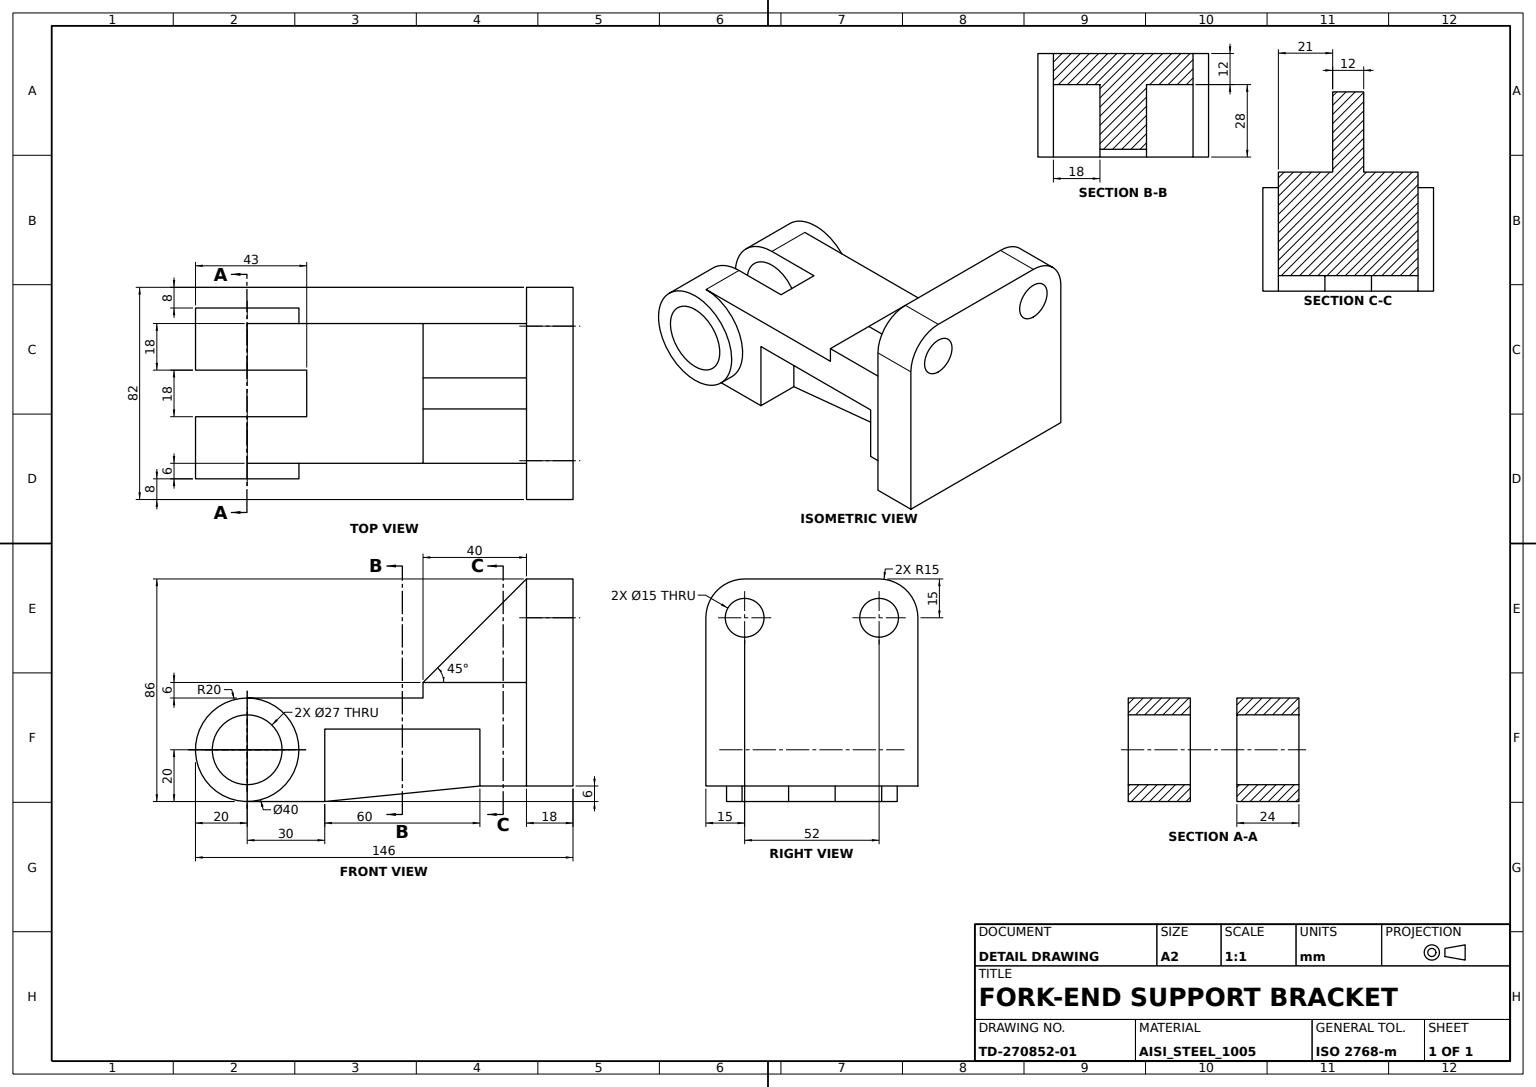
ISO-10303-21;
HEADER;
FILE_DESCRIPTION((''),'2;1');
FILE_NAME('','',(''),(''),'','','');
FILE_SCHEMA(('AUTOMOTIVE_DESIGN'));
ENDSEC;
DATA;
#1=APPLICATION_CONTEXT('');
#2=PRODUCT_CONTEXT('',#1,'mechanical');
#3=PRODUCT('','','',(#2));
#4=PRODUCT_DEFINITION_FORMATION('','',#3);
#5=PRODUCT_DEFINITION_CONTEXT('',#1,'design');
#6=PRODUCT_DEFINITION('','',#4,#5);
#7=PRODUCT_DEFINITION_SHAPE('','',#6);
#8=(LENGTH_UNIT()NAMED_UNIT(*)SI_UNIT(.MILLI.,.METRE.));
#9=(NAMED_UNIT(*)PLANE_ANGLE_UNIT()SI_UNIT($,.RADIAN.));
#10=(NAMED_UNIT(*)SI_UNIT($,.STERADIAN.)SOLID_ANGLE_UNIT());
#11=UNCERTAINTY_MEASURE_WITH_UNIT(LENGTH_MEASURE(0.005),#8,'distance_accuracy_value','');
#12=(GEOMETRIC_REPRESENTATION_CONTEXT(3)GLOBAL_UNCERTAINTY_ASSIGNED_CONTEXT((#11))GLOBAL_UNIT_ASSIGNED_CONTEXT((#8,#9,#10))REPRESENTATION_CONTEXT('',''));
#13=CARTESIAN_POINT('',(9.,-96.,-46.));
#14=VERTEX_POINT('',#13);
#15=CARTESIAN_POINT('',(-9.,-96.,-46.));
#16=VERTEX_POINT('',#15);
#17=DIRECTION('',(-1.,0.,0.));
#18=VECTOR('',#17,1000.);
#19=LINE('',#13,#18);
#20=EDGE_CURVE('',#14,#16,#19,.T.);
#21=ORIENTED_EDGE('',*,*,#20,.F.);
#22=CARTESIAN_POINT('',(27.,-96.,-46.));
#23=VERTEX_POINT('',#22);
#24=LINE('',#22,#18);
#25=EDGE_CURVE('',#23,#14,#24,.T.);
#26=ORIENTED_EDGE('',*,*,#25,.F.);
#27=CARTESIAN_POINT('',(27.,-126.,-46.));
#28=VERTEX_POINT('',#27);
#29=DIRECTION('',(0.,1.,0.));
#30=VECTOR('',#29,1000.);
#31=LINE('',#27,#30);
#32=EDGE_CURVE('',#28,#23,#31,.T.);
#33=ORIENTED_EDGE('',*,*,#32,.F.);
#34=CARTESIAN_POINT('',(9.,-126.,-46.));
#35=VERTEX_POINT('',#34);
#36=LINE('',#27,#18);
#37=EDGE_CURVE('',#28,#35,#36,.T.);
#38=ORIENTED_EDGE('',*,*,#37,.T.);
#39=CARTESIAN_POINT('',(9.,-103.,-46.));
#40=VERTEX_POINT('',#39);
#41=DIRECTION('',(0.,-1.,0.));
#42=VECTOR('',#41,1000.);
#43=LINE('',#34,#42);
#44=EDGE_CURVE('',#40,#35,#43,.T.);
#45=ORIENTED_EDGE('',*,*,#44,.F.);
#46=CARTESIAN_POINT('',(-9.,-103.,-46.));
#47=VERTEX_POINT('',#46);
#48=CARTESIAN_POINT('',(27.,-103.,-46.));
#49=DIRECTION('',(1.,0.,0.));
#50=VECTOR('',#49,1000.);
#51=LINE('',#48,#50);
#52=EDGE_CURVE('',#47,#40,#51,.T.);
#53=ORIENTED_EDGE('',*,*,#52,.F.);
#54=CARTESIAN_POINT('',(-9.,-126.,-46.));
#55=VERTEX_POINT('',#54);
#56=LINE('',#54,#30);
#57=EDGE_CURVE('',#55,#47,#56,.T.);
#58=ORIENTED_EDGE('',*,*,#57,.F.);
#59=CARTESIAN_POINT('',(-27.,-126.,-46.));
#60=VERTEX_POINT('',#59);
#61=EDGE_CURVE('',#55,#60,#36,.T.);
#62=ORIENTED_EDGE('',*,*,#61,.T.);
#63=CARTESIAN_POINT('',(-27.,-96.,-46.));
#64=VERTEX_POINT('',#63);
#65=LINE('',#59,#30);
#66=EDGE_CURVE('',#60,#64,#65,.T.);
#67=ORIENTED_EDGE('',*,*,#66,.T.);
#68=EDGE_CURVE('',#16,#64,#24,.T.);
#69=ORIENTED_EDGE('',*,*,#68,.F.);
#70=EDGE_LOOP('',(#21,#26,#33,#38,#45,#53,#58,#62,#67,#69));
#71=FACE_BOUND('',#70,.T.);
#72=DIRECTION('',(0.,0.,1.));
#73=AXIS2_PLACEMENT_3D('',#27,#72,#41);
#74=PLANE('',#73);
#75=ADVANCED_FACE('',(#71),#74,.F.);
#76=CARTESIAN_POINT('',(-6.,-18.,40.));
#77=VERTEX_POINT('',#76);
#78=CARTESIAN_POINT('',(-6.,-18.,0.));
#79=VERTEX_POINT('',#78);
#80=DIRECTION('',(0.,0.,-1.));
#81=VECTOR('',#80,1000.);
#82=LINE('',#76,#81);
#83=EDGE_CURVE('',#77,#79,#82,.T.);
#84=ORIENTED_EDGE('',*,*,#83,.T.);
#85=CARTESIAN_POINT('',(-6.,-58.,0.));
#86=VERTEX_POINT('',#85);
#87=LINE('',#78,#42);
#88=EDGE_CURVE('',#79,#86,#87,.T.);
#89=ORIENTED_EDGE('',*,*,#88,.T.);
#90=DIRECTION('',(0.,0.707106781,0.707106781));
#91=VECTOR('',#90,1000.);
#92=LINE('',#85,#91);
#93=EDGE_CURVE('',#86,#77,#92,.T.);
#94=ORIENTED_EDGE('',*,*,#93,.T.);
#95=EDGE_LOOP('',(#84,#89,#94));
#96=FACE_BOUND('',#95,.T.);
#97=CARTESIAN_POINT('',(-6.,0.,0.));
#98=AXIS2_PLACEMENT_3D('',#97,#17,#72);
#99=PLANE('',#98);
#100=ADVANCED_FACE('',(#96),#99,.T.);
#101=CARTESIAN_POINT('',(-9.,-36.,-18.));
#102=VERTEX_POINT('',#101);
#103=CARTESIAN_POINT('',(-9.,-36.,-40.));
#104=VERTEX_POINT('',#103);
#105=LINE('',#101,#81);
#106=EDGE_CURVE('',#102,#104,#105,.T.);
#107=ORIENTED_EDGE('',*,*,#106,.F.);
#108=CARTESIAN_POINT('',(-27.,-36.,-18.));
#109=VERTEX_POINT('',#108);
#110=CARTESIAN_POINT('',(47.,-36.,-18.));
#111=LINE('',#110,#18);
#112=EDGE_CURVE('',#109,#102,#111,.F.);
#113=ORIENTED_EDGE('',*,*,#112,.F.);
#114=CARTESIAN_POINT('',(-27.,-36.,-40.));
#115=VERTEX_POINT('',#114);
#116=CARTESIAN_POINT('',(-27.,-36.,0.));
#117=VECTOR('',#72,1000.);
#118=LINE('',#116,#117);
#119=EDGE_CURVE('',#115,#109,#118,.T.);
#120=ORIENTED_EDGE('',*,*,#119,.F.);
#121=CARTESIAN_POINT('',(27.,-36.,-40.));
#122=LINE('',#121,#18);
#123=EDGE_CURVE('',#104,#115,#122,.T.);
#124=ORIENTED_EDGE('',*,*,#123,.F.);
#125=EDGE_LOOP('',(#107,#113,#120,#124));
#126=FACE_BOUND('',#125,.T.);
#127=CARTESIAN_POINT('',(47.,-36.,-57.));
#128=AXIS2_PLACEMENT_3D('',#127,#41,#80);
#129=PLANE('',#128);
#130=ADVANCED_FACE('',(#126),#129,.T.);
#131=ORIENTED_EDGE('',*,*,#123,.T.);
#132=CARTESIAN_POINT('',(-27.,-18.,-40.));
#133=VERTEX_POINT('',#132);
#134=LINE('',#132,#42);
#135=EDGE_CURVE('',#133,#115,#134,.T.);
#136=ORIENTED_EDGE('',*,*,#135,.F.);
#137=CARTESIAN_POINT('',(-41.,-18.,-40.));
#138=VERTEX_POINT('',#137);
#139=LINE('',#137,#50);
#140=EDGE_CURVE('',#138,#133,#139,.T.);
#141=ORIENTED_EDGE('',*,*,#140,.F.);
#142=CARTESIAN_POINT('',(-41.,0.,-40.));
#143=VERTEX_POINT('',#142);
#144=LINE('',#137,#30);
#145=EDGE_CURVE('',#138,#143,#144,.T.);
#146=ORIENTED_EDGE('',*,*,#145,.T.);
#147=CARTESIAN_POINT('',(41.,0.,-40.));
#148=VERTEX_POINT('',#147);
#149=LINE('',#142,#50);
#150=EDGE_CURVE('',#143,#148,#149,.T.);
#151=ORIENTED_EDGE('',*,*,#150,.T.);
#152=CARTESIAN_POINT('',(41.,-18.,-40.));
#153=VERTEX_POINT('',#152);
#154=LINE('',#152,#30);
#155=EDGE_CURVE('',#153,#148,#154,.T.);
#156=ORIENTED_EDGE('',*,*,#155,.F.);
#157=CARTESIAN_POINT('',(27.,-18.,-40.));
#158=VERTEX_POINT('',#157);
#159=EDGE_CURVE('',#158,#153,#139,.T.);
#160=ORIENTED_EDGE('',*,*,#159,.F.);
#161=VERTEX_POINT('',#121);
#162=LINE('',#157,#42);
#163=EDGE_CURVE('',#158,#161,#162,.T.);
#164=ORIENTED_EDGE('',*,*,#163,.T.);
#165=CARTESIAN_POINT('',(9.,-36.,-40.));
#166=VERTEX_POINT('',#165);
#167=EDGE_CURVE('',#161,#166,#122,.T.);
#168=ORIENTED_EDGE('',*,*,#167,.T.);
#169=LINE('',#165,#18);
#170=EDGE_CURVE('',#166,#104,#169,.T.);
#171=ORIENTED_EDGE('',*,*,#170,.T.);
#172=EDGE_LOOP('',(#131,#136,#141,#146,#151,#156,#160,#164,#168,#171));
#173=FACE_BOUND('',#172,.T.);
#174=AXIS2_PLACEMENT_3D('',#157,#80,#29);
#175=PLANE('',#174);
#176=ADVANCED_FACE('',(#173),#175,.T.);
#177=ORIENTED_EDGE('',*,*,#37,.F.);
#178=CARTESIAN_POINT('',(27.,-126.,-6.));
#179=VERTEX_POINT('',#178);
#180=CARTESIAN_POINT('',(27.,-126.,-26.));
#181=AXIS2_PLACEMENT_3D('',#180,#17,#72);
#182=CIRCLE('',#181,20.);
#183=EDGE_CURVE('',#28,#179,#182,.F.);
#184=ORIENTED_EDGE('',*,*,#183,.T.);
#185=CARTESIAN_POINT('',(9.,-126.,-6.));
#186=VERTEX_POINT('',#185);
#187=LINE('',#178,#18);
#188=EDGE_CURVE('',#179,#186,#187,.T.);
#189=ORIENTED_EDGE('',*,*,#188,.T.);
#190=CARTESIAN_POINT('',(9.,-126.,-26.));
#191=AXIS2_PLACEMENT_3D('',#190,#17,#41);
#192=CIRCLE('',#191,20.);
#193=EDGE_CURVE('',#35,#186,#192,.T.);
#194=ORIENTED_EDGE('',*,*,#193,.F.);
#195=EDGE_LOOP('',(#177,#184,#189,#194));
#196=FACE_BOUND('',#195,.T.);
#197=CARTESIAN_POINT('',(33.,-106.,-26.));
#198=VERTEX_POINT('',#197);
#199=CARTESIAN_POINT('',(33.,-126.,-26.));
#200=AXIS2_PLACEMENT_3D('',#199,#49,#29);
#201=CIRCLE('',#200,20.);
#202=EDGE_CURVE('',#198,#198,#201,.T.);
#203=ORIENTED_EDGE('',*,*,#202,.F.);
#204=EDGE_LOOP('',(#203));
#205=FACE_BOUND('',#204,.T.);
#206=AXIS2_PLACEMENT_3D('',#199,#17,#72);
#207=CYLINDRICAL_SURFACE('',#206,20.);
#208=ADVANCED_FACE('',(#196,#205),#207,.T.);
#209=CARTESIAN_POINT('',(9.,-96.,-18.));
#210=VERTEX_POINT('',#209);
#211=LINE('',#13,#117);
#212=EDGE_CURVE('',#14,#210,#211,.T.);
#213=ORIENTED_EDGE('',*,*,#212,.F.);
#214=DIRECTION('',(0.,-0.99503719,-0.099503719));
#215=VECTOR('',#214,1000.);
#216=LINE('',#165,#215);
#217=EDGE_CURVE('',#166,#14,#216,.T.);
#218=ORIENTED_EDGE('',*,*,#217,.F.);
#219=CARTESIAN_POINT('',(9.,-36.,-18.));
#220=VERTEX_POINT('',#219);
#221=LINE('',#219,#81);
#222=EDGE_CURVE('',#220,#166,#221,.T.);
#223=ORIENTED_EDGE('',*,*,#222,.F.);
#224=LINE('',#209,#30);
#225=EDGE_CURVE('',#210,#220,#224,.T.);
#226=ORIENTED_EDGE('',*,*,#225,.F.);
#227=EDGE_LOOP('',(#213,#218,#223,#226));
#228=FACE_BOUND('',#227,.T.);
#229=CARTESIAN_POINT('',(9.,0.,0.));
#230=AXIS2_PLACEMENT_3D('',#229,#17,#72);
#231=PLANE('',#230);
#232=ADVANCED_FACE('',(#228),#231,.F.);
#233=CARTESIAN_POINT('',(-26.,-18.,32.5));
#234=VERTEX_POINT('',#233);
#235=CARTESIAN_POINT('',(-26.,-18.,25.));
#236=AXIS2_PLACEMENT_3D('',#235,#29,#72);
#237=CIRCLE('',#236,7.5);
#238=EDGE_CURVE('',#234,#234,#237,.T.);
#239=ORIENTED_EDGE('',*,*,#238,.T.);
#240=EDGE_LOOP('',(#239));
#241=FACE_BOUND('',#240,.T.);
#242=ORIENTED_EDGE('',*,*,#140,.T.);
#243=CARTESIAN_POINT('',(-27.,-18.,0.));
#244=VERTEX_POINT('',#243);
#245=LINE('',#243,#81);
#246=EDGE_CURVE('',#244,#133,#245,.T.);
#247=ORIENTED_EDGE('',*,*,#246,.F.);
#248=CARTESIAN_POINT('',(27.,-18.,0.));
#249=LINE('',#248,#18);
#250=EDGE_CURVE('',#79,#244,#249,.T.);
#251=ORIENTED_EDGE('',*,*,#250,.F.);
#252=ORIENTED_EDGE('',*,*,#83,.F.);
#253=CARTESIAN_POINT('',(-26.,-18.,40.));
#254=VERTEX_POINT('',#253);
#255=CARTESIAN_POINT('',(26.,-18.,40.));
#256=LINE('',#255,#18);
#257=EDGE_CURVE('',#77,#254,#256,.T.);
#258=ORIENTED_EDGE('',*,*,#257,.T.);
#259=CARTESIAN_POINT('',(-41.,-18.,25.));
#260=VERTEX_POINT('',#259);
#261=AXIS2_PLACEMENT_3D('',#235,#41,#49);
#262=CIRCLE('',#261,15.);
#263=EDGE_CURVE('',#254,#260,#262,.T.);
#264=ORIENTED_EDGE('',*,*,#263,.T.);
#265=LINE('',#259,#81);
#266=EDGE_CURVE('',#260,#138,#265,.T.);
#267=ORIENTED_EDGE('',*,*,#266,.T.);
#268=EDGE_LOOP('',(#242,#247,#251,#252,#258,#264,#267));
#269=FACE_BOUND('',#268,.T.);
#270=CARTESIAN_POINT('',(26.,-18.,25.));
#271=AXIS2_PLACEMENT_3D('',#270,#41,#80);
#272=PLANE('',#271);
#273=ADVANCED_FACE('',(#241,#269),#272,.T.);
#274=CARTESIAN_POINT('',(9.,-139.5,-26.));
#275=VERTEX_POINT('',#274);
#276=CIRCLE('',#191,13.5);
#277=EDGE_CURVE('',#275,#275,#276,.F.);
#278=ORIENTED_EDGE('',*,*,#277,.F.);
#279=EDGE_LOOP('',(#278));
#280=FACE_BOUND('',#279,.T.);
#281=CARTESIAN_POINT('',(33.,-126.,-12.5));
#282=VERTEX_POINT('',#281);
#283=CIRCLE('',#206,13.5);
#284=EDGE_CURVE('',#282,#282,#283,.T.);
#285=ORIENTED_EDGE('',*,*,#284,.F.);
#286=EDGE_LOOP('',(#285));
#287=FACE_BOUND('',#286,.T.);
#288=CYLINDRICAL_SURFACE('',#206,13.5);
#289=ADVANCED_FACE('',(#280,#287),#288,.F.);
#290=ORIENTED_EDGE('',*,*,#225,.T.);
#291=CARTESIAN_POINT('',(27.,-36.,-18.));
#292=VERTEX_POINT('',#291);
#293=EDGE_CURVE('',#220,#292,#111,.F.);
#294=ORIENTED_EDGE('',*,*,#293,.T.);
#295=CARTESIAN_POINT('',(27.,-96.,-18.));
#296=VERTEX_POINT('',#295);
#297=CARTESIAN_POINT('',(27.,0.,-18.));
#298=LINE('',#297,#42);
#299=EDGE_CURVE('',#292,#296,#298,.T.);
#300=ORIENTED_EDGE('',*,*,#299,.T.);
#301=CARTESIAN_POINT('',(47.,-96.,-18.));
#302=LINE('',#301,#18);
#303=EDGE_CURVE('',#210,#296,#302,.F.);
#304=ORIENTED_EDGE('',*,*,#303,.F.);
#305=EDGE_LOOP('',(#290,#294,#300,#304));
#306=FACE_BOUND('',#305,.T.);
#307=AXIS2_PLACEMENT_3D('',#110,#80,#29);
#308=PLANE('',#307);
#309=ADVANCED_FACE('',(#306),#308,.T.);
#310=ORIENTED_EDGE('',*,*,#263,.F.);
#311=CARTESIAN_POINT('',(-26.,0.,40.));
#312=VERTEX_POINT('',#311);
#313=LINE('',#253,#30);
#314=EDGE_CURVE('',#254,#312,#313,.T.);
#315=ORIENTED_EDGE('',*,*,#314,.T.);
#316=CARTESIAN_POINT('',(-41.,0.,25.));
#317=VERTEX_POINT('',#316);
#318=CARTESIAN_POINT('',(-26.,0.,25.));
#319=AXIS2_PLACEMENT_3D('',#318,#41,#49);
#320=CIRCLE('',#319,15.);
#321=EDGE_CURVE('',#312,#317,#320,.T.);
#322=ORIENTED_EDGE('',*,*,#321,.T.);
#323=LINE('',#259,#30);
#324=EDGE_CURVE('',#260,#317,#323,.T.);
#325=ORIENTED_EDGE('',*,*,#324,.F.);
#326=EDGE_LOOP('',(#310,#315,#322,#325));
#327=FACE_BOUND('',#326,.T.);
#328=CYLINDRICAL_SURFACE('',#236,15.);
#329=ADVANCED_FACE('',(#327),#328,.T.);
#330=ORIENTED_EDGE('',*,*,#20,.T.);
#331=LINE('',#103,#215);
#332=EDGE_CURVE('',#104,#16,#331,.T.);
#333=ORIENTED_EDGE('',*,*,#332,.F.);
#334=ORIENTED_EDGE('',*,*,#170,.F.);
#335=ORIENTED_EDGE('',*,*,#217,.T.);
#336=EDGE_LOOP('',(#330,#333,#334,#335));
#337=FACE_BOUND('',#336,.T.);
#338=DIRECTION('',(0.,0.099503719,-0.99503719));
#339=DIRECTION('',(0.,0.99503719,0.099503719));
#340=AXIS2_PLACEMENT_3D('',#165,#338,#339);
#341=PLANE('',#340);
#342=ADVANCED_FACE('',(#337),#341,.T.);
#343=CARTESIAN_POINT('',(-9.,-112.5,-26.));
#344=VERTEX_POINT('',#343);
#345=CARTESIAN_POINT('',(-9.,-126.,-26.));
#346=AXIS2_PLACEMENT_3D('',#345,#49,#29);
#347=CIRCLE('',#346,13.5);
#348=EDGE_CURVE('',#344,#344,#347,.F.);
#349=ORIENTED_EDGE('',*,*,#348,.F.);
#350=EDGE_LOOP('',(#349));
#351=FACE_BOUND('',#350,.T.);
#352=CARTESIAN_POINT('',(-33.,-126.,-39.5));
#353=VERTEX_POINT('',#352);
#354=CARTESIAN_POINT('',(-33.,-126.,-26.));
#355=AXIS2_PLACEMENT_3D('',#354,#49,#80);
#356=CIRCLE('',#355,13.5);
#357=EDGE_CURVE('',#353,#353,#356,.T.);
#358=ORIENTED_EDGE('',*,*,#357,.F.);
#359=EDGE_LOOP('',(#358));
#360=FACE_BOUND('',#359,.T.);
#361=ADVANCED_FACE('',(#351,#360),#288,.F.);
#362=ORIENTED_EDGE('',*,*,#357,.T.);
#363=EDGE_LOOP('',(#362));
#364=FACE_BOUND('',#363,.T.);
#365=CARTESIAN_POINT('',(-33.,-106.,-26.));
#366=VERTEX_POINT('',#365);
#367=AXIS2_PLACEMENT_3D('',#354,#49,#29);
#368=CIRCLE('',#367,20.);
#369=EDGE_CURVE('',#366,#366,#368,.T.);
#370=ORIENTED_EDGE('',*,*,#369,.F.);
#371=EDGE_LOOP('',(#370));
#372=FACE_BOUND('',#371,.T.);
#373=PLANE('',#355);
#374=ADVANCED_FACE('',(#364,#372),#373,.F.);
#375=ORIENTED_EDGE('',*,*,#183,.F.);
#376=ORIENTED_EDGE('',*,*,#32,.T.);
#377=CARTESIAN_POINT('',(27.,-96.,0.));
#378=LINE('',#377,#81);
#379=EDGE_CURVE('',#296,#23,#378,.T.);
#380=ORIENTED_EDGE('',*,*,#379,.F.);
#381=ORIENTED_EDGE('',*,*,#299,.F.);
#382=CARTESIAN_POINT('',(27.,-36.,0.));
#383=LINE('',#382,#117);
#384=EDGE_CURVE('',#161,#292,#383,.T.);
#385=ORIENTED_EDGE('',*,*,#384,.F.);
#386=ORIENTED_EDGE('',*,*,#163,.F.);
#387=VERTEX_POINT('',#248);
#388=LINE('',#248,#81);
#389=EDGE_CURVE('',#387,#158,#388,.T.);
#390=ORIENTED_EDGE('',*,*,#389,.F.);
#391=CARTESIAN_POINT('',(27.,-58.,0.));
#392=VERTEX_POINT('',#391);
#393=CARTESIAN_POINT('',(27.,-126.,0.));
#394=LINE('',#393,#30);
#395=EDGE_CURVE('',#392,#387,#394,.T.);
#396=ORIENTED_EDGE('',*,*,#395,.F.);
#397=CARTESIAN_POINT('',(27.,-58.,-6.));
#398=VERTEX_POINT('',#397);
#399=LINE('',#391,#117);
#400=EDGE_CURVE('',#398,#392,#399,.T.);
#401=ORIENTED_EDGE('',*,*,#400,.F.);
#402=CARTESIAN_POINT('',(27.,0.,-6.));
#403=LINE('',#402,#30);
#404=EDGE_CURVE('',#179,#398,#403,.T.);
#405=ORIENTED_EDGE('',*,*,#404,.F.);
#406=EDGE_LOOP('',(#375,#376,#380,#381,#385,#386,#390,#396,#401,#405));
#407=FACE_BOUND('',#406,.T.);
#408=CARTESIAN_POINT('',(27.,0.,0.));
#409=AXIS2_PLACEMENT_3D('',#408,#17,#72);
#410=PLANE('',#409);
#411=ADVANCED_FACE('',(#407),#410,.F.);
#412=ORIENTED_EDGE('',*,*,#52,.T.);
#413=CARTESIAN_POINT('',(9.,-103.,-6.));
#414=VERTEX_POINT('',#413);
#415=CARTESIAN_POINT('',(9.,-103.,34.));
#416=LINE('',#415,#81);
#417=EDGE_CURVE('',#40,#414,#416,.F.);
#418=ORIENTED_EDGE('',*,*,#417,.T.);
#419=CARTESIAN_POINT('',(-9.,-103.,-6.));
#420=VERTEX_POINT('',#419);
#421=CARTESIAN_POINT('',(47.,-103.,-6.));
#422=LINE('',#421,#50);
#423=EDGE_CURVE('',#420,#414,#422,.T.);
#424=ORIENTED_EDGE('',*,*,#423,.F.);
#425=CARTESIAN_POINT('',(-9.,-103.,34.));
#426=LINE('',#425,#81);
#427=EDGE_CURVE('',#47,#420,#426,.F.);
#428=ORIENTED_EDGE('',*,*,#427,.F.);
#429=EDGE_LOOP('',(#412,#418,#424,#428));
#430=FACE_BOUND('',#429,.T.);
#431=AXIS2_PLACEMENT_3D('',#415,#41,#80);
#432=PLANE('',#431);
#433=ADVANCED_FACE('',(#430),#432,.T.);
#434=CARTESIAN_POINT('',(-9.,-126.,-6.));
#435=VERTEX_POINT('',#434);
#436=CARTESIAN_POINT('',(-9.,-133.,-6.));
#437=LINE('',#436,#30);
#438=EDGE_CURVE('',#435,#420,#437,.T.);
#439=ORIENTED_EDGE('',*,*,#438,.F.);
#440=CIRCLE('',#346,20.);
#441=EDGE_CURVE('',#435,#55,#440,.T.);
#442=ORIENTED_EDGE('',*,*,#441,.T.);
#443=ORIENTED_EDGE('',*,*,#57,.T.);
#444=ORIENTED_EDGE('',*,*,#427,.T.);
#445=EDGE_LOOP('',(#439,#442,#443,#444));
#446=FACE_BOUND('',#445,.T.);
#447=ORIENTED_EDGE('',*,*,#348,.T.);
#448=EDGE_LOOP('',(#447));
#449=FACE_BOUND('',#448,.T.);
#450=AXIS2_PLACEMENT_3D('',#425,#49,#29);
#451=PLANE('',#450);
#452=ADVANCED_FACE('',(#446,#449),#451,.T.);
#453=ORIENTED_EDGE('',*,*,#238,.F.);
#454=EDGE_LOOP('',(#453));
#455=FACE_BOUND('',#454,.T.);
#456=CARTESIAN_POINT('',(-26.,0.,17.5));
#457=VERTEX_POINT('',#456);
#458=AXIS2_PLACEMENT_3D('',#318,#41,#80);
#459=CIRCLE('',#458,7.5);
#460=EDGE_CURVE('',#457,#457,#459,.T.);
#461=ORIENTED_EDGE('',*,*,#460,.F.);
#462=EDGE_LOOP('',(#461));
#463=FACE_BOUND('',#462,.T.);
#464=CYLINDRICAL_SURFACE('',#236,7.5);
#465=ADVANCED_FACE('',(#455,#463),#464,.F.);
#466=ORIENTED_EDGE('',*,*,#277,.T.);
#467=EDGE_LOOP('',(#466));
#468=FACE_BOUND('',#467,.T.);
#469=ORIENTED_EDGE('',*,*,#193,.T.);
#470=CARTESIAN_POINT('',(9.,-133.,-6.));
#471=LINE('',#470,#42);
#472=EDGE_CURVE('',#414,#186,#471,.T.);
#473=ORIENTED_EDGE('',*,*,#472,.F.);
#474=ORIENTED_EDGE('',*,*,#417,.F.);
#475=ORIENTED_EDGE('',*,*,#44,.T.);
#476=EDGE_LOOP('',(#469,#473,#474,#475));
#477=FACE_BOUND('',#476,.T.);
#478=CARTESIAN_POINT('',(9.,-183.,34.));
#479=AXIS2_PLACEMENT_3D('',#478,#17,#41);
#480=PLANE('',#479);
#481=ADVANCED_FACE('',(#468,#477),#480,.T.);
#482=ORIENTED_EDGE('',*,*,#93,.F.);
#483=CARTESIAN_POINT('',(6.,-58.,0.));
#484=VERTEX_POINT('',#483);
#485=LINE('',#483,#18);
#486=EDGE_CURVE('',#484,#86,#485,.T.);
#487=ORIENTED_EDGE('',*,*,#486,.F.);
#488=CARTESIAN_POINT('',(6.,-18.,40.));
#489=VERTEX_POINT('',#488);
#490=LINE('',#483,#91);
#491=EDGE_CURVE('',#484,#489,#490,.T.);
#492=ORIENTED_EDGE('',*,*,#491,.T.);
#493=LINE('',#488,#18);
#494=EDGE_CURVE('',#489,#77,#493,.T.);
#495=ORIENTED_EDGE('',*,*,#494,.T.);
#496=EDGE_LOOP('',(#482,#487,#492,#495));
#497=FACE_BOUND('',#496,.T.);
#498=DIRECTION('',(0.,-0.707106781,0.707106781));
#499=DIRECTION('',(0.,-0.707106781,-0.707106781));
#500=AXIS2_PLACEMENT_3D('',#483,#498,#499);
#501=PLANE('',#500);
#502=ADVANCED_FACE('',(#497),#501,.T.);
#503=CARTESIAN_POINT('',(-27.,-96.,-18.));
#504=VERTEX_POINT('',#503);
#505=CARTESIAN_POINT('',(-27.,-96.,0.));
#506=LINE('',#505,#81);
#507=EDGE_CURVE('',#504,#64,#506,.T.);
#508=ORIENTED_EDGE('',*,*,#507,.F.);
#509=CARTESIAN_POINT('',(-9.,-96.,-18.));
#510=VERTEX_POINT('',#509);
#511=EDGE_CURVE('',#504,#510,#302,.F.);
#512=ORIENTED_EDGE('',*,*,#511,.T.);
#513=LINE('',#15,#117);
#514=EDGE_CURVE('',#16,#510,#513,.T.);
#515=ORIENTED_EDGE('',*,*,#514,.F.);
#516=ORIENTED_EDGE('',*,*,#68,.T.);
#517=EDGE_LOOP('',(#508,#512,#515,#516));
#518=FACE_BOUND('',#517,.T.);
#519=AXIS2_PLACEMENT_3D('',#301,#29,#72);
#520=PLANE('',#519);
#521=ADVANCED_FACE('',(#518),#520,.T.);
#522=ORIENTED_EDGE('',*,*,#202,.T.);
#523=EDGE_LOOP('',(#522));
#524=FACE_BOUND('',#523,.T.);
#525=ORIENTED_EDGE('',*,*,#284,.T.);
#526=EDGE_LOOP('',(#525));
#527=FACE_BOUND('',#526,.T.);
#528=AXIS2_PLACEMENT_3D('',#199,#49,#80);
#529=PLANE('',#528);
#530=ADVANCED_FACE('',(#524,#527),#529,.T.);
#531=ORIENTED_EDGE('',*,*,#257,.F.);
#532=ORIENTED_EDGE('',*,*,#494,.F.);
#533=VERTEX_POINT('',#255);
#534=EDGE_CURVE('',#533,#489,#256,.T.);
#535=ORIENTED_EDGE('',*,*,#534,.F.);
#536=CARTESIAN_POINT('',(26.,0.,40.));
#537=VERTEX_POINT('',#536);
#538=LINE('',#255,#30);
#539=EDGE_CURVE('',#533,#537,#538,.T.);
#540=ORIENTED_EDGE('',*,*,#539,.T.);
#541=LINE('',#536,#18);
#542=EDGE_CURVE('',#537,#312,#541,.T.);
#543=ORIENTED_EDGE('',*,*,#542,.T.);
#544=ORIENTED_EDGE('',*,*,#314,.F.);
#545=EDGE_LOOP('',(#531,#532,#535,#540,#543,#544));
#546=FACE_BOUND('',#545,.T.);
#547=AXIS2_PLACEMENT_3D('',#255,#80,#17);
#548=PLANE('',#547);
#549=ADVANCED_FACE('',(#546),#548,.F.);
#550=CARTESIAN_POINT('',(26.,0.,17.5));
#551=VERTEX_POINT('',#550);
#552=CARTESIAN_POINT('',(26.,0.,25.));
#553=AXIS2_PLACEMENT_3D('',#552,#41,#80);
#554=CIRCLE('',#553,7.5);
#555=EDGE_CURVE('',#551,#551,#554,.T.);
#556=ORIENTED_EDGE('',*,*,#555,.F.);
#557=EDGE_LOOP('',(#556));
#558=FACE_BOUND('',#557,.T.);
#559=CARTESIAN_POINT('',(26.,-18.,32.5));
#560=VERTEX_POINT('',#559);
#561=AXIS2_PLACEMENT_3D('',#270,#29,#72);
#562=CIRCLE('',#561,7.5);
#563=EDGE_CURVE('',#560,#560,#562,.T.);
#564=ORIENTED_EDGE('',*,*,#563,.F.);
#565=EDGE_LOOP('',(#564));
#566=FACE_BOUND('',#565,.T.);
#567=CYLINDRICAL_SURFACE('',#561,7.5);
#568=ADVANCED_FACE('',(#558,#566),#567,.F.);
#569=ORIENTED_EDGE('',*,*,#303,.T.);
#570=ORIENTED_EDGE('',*,*,#379,.T.);
#571=ORIENTED_EDGE('',*,*,#25,.T.);
#572=ORIENTED_EDGE('',*,*,#212,.T.);
#573=EDGE_LOOP('',(#569,#570,#571,#572));
#574=FACE_BOUND('',#573,.T.);
#575=ADVANCED_FACE('',(#574),#520,.T.);
#576=ORIENTED_EDGE('',*,*,#369,.T.);
#577=EDGE_LOOP('',(#576));
#578=FACE_BOUND('',#577,.T.);
#579=CARTESIAN_POINT('',(-27.,-126.,-6.));
#580=VERTEX_POINT('',#579);
#581=CARTESIAN_POINT('',(-27.,-126.,-26.));
#582=AXIS2_PLACEMENT_3D('',#581,#17,#72);
#583=CIRCLE('',#582,20.);
#584=EDGE_CURVE('',#60,#580,#583,.F.);
#585=ORIENTED_EDGE('',*,*,#584,.F.);
#586=ORIENTED_EDGE('',*,*,#61,.F.);
#587=ORIENTED_EDGE('',*,*,#441,.F.);
#588=EDGE_CURVE('',#435,#580,#187,.T.);
#589=ORIENTED_EDGE('',*,*,#588,.T.);
#590=EDGE_LOOP('',(#585,#586,#587,#589));
#591=FACE_BOUND('',#590,.T.);
#592=ADVANCED_FACE('',(#578,#591),#207,.T.);
#593=ORIENTED_EDGE('',*,*,#400,.T.);
#594=CARTESIAN_POINT('',(47.,-58.,0.));
#595=LINE('',#594,#18);
#596=EDGE_CURVE('',#392,#484,#595,.T.);
#597=ORIENTED_EDGE('',*,*,#596,.T.);
#598=ORIENTED_EDGE('',*,*,#486,.T.);
#599=CARTESIAN_POINT('',(-27.,-58.,0.));
#600=VERTEX_POINT('',#599);
#601=EDGE_CURVE('',#86,#600,#595,.T.);
#602=ORIENTED_EDGE('',*,*,#601,.T.);
#603=CARTESIAN_POINT('',(-27.,-58.,-6.));
#604=VERTEX_POINT('',#603);
#605=LINE('',#599,#117);
#606=EDGE_CURVE('',#604,#600,#605,.T.);
#607=ORIENTED_EDGE('',*,*,#606,.F.);
#608=CARTESIAN_POINT('',(47.,-58.,-6.));
#609=LINE('',#608,#18);
#610=EDGE_CURVE('',#604,#398,#609,.F.);
#611=ORIENTED_EDGE('',*,*,#610,.T.);
#612=EDGE_LOOP('',(#593,#597,#598,#602,#607,#611));
#613=FACE_BOUND('',#612,.T.);
#614=AXIS2_PLACEMENT_3D('',#608,#41,#80);
#615=PLANE('',#614);
#616=ADVANCED_FACE('',(#613),#615,.T.);
#617=LINE('',#509,#30);
#618=EDGE_CURVE('',#510,#102,#617,.T.);
#619=ORIENTED_EDGE('',*,*,#618,.F.);
#620=ORIENTED_EDGE('',*,*,#511,.F.);
#621=CARTESIAN_POINT('',(-27.,0.,-18.));
#622=LINE('',#621,#42);
#623=EDGE_CURVE('',#109,#504,#622,.T.);
#624=ORIENTED_EDGE('',*,*,#623,.F.);
#625=ORIENTED_EDGE('',*,*,#112,.T.);
#626=EDGE_LOOP('',(#619,#620,#624,#625));
#627=FACE_BOUND('',#626,.T.);
#628=ADVANCED_FACE('',(#627),#308,.T.);
#629=ORIENTED_EDGE('',*,*,#618,.T.);
#630=ORIENTED_EDGE('',*,*,#106,.T.);
#631=ORIENTED_EDGE('',*,*,#332,.T.);
#632=ORIENTED_EDGE('',*,*,#514,.T.);
#633=EDGE_LOOP('',(#629,#630,#631,#632));
#634=FACE_BOUND('',#633,.T.);
#635=CARTESIAN_POINT('',(-9.,0.,0.));
#636=AXIS2_PLACEMENT_3D('',#635,#17,#72);
#637=PLANE('',#636);
#638=ADVANCED_FACE('',(#634),#637,.T.);
#639=ORIENTED_EDGE('',*,*,#250,.T.);
#640=CARTESIAN_POINT('',(-27.,-126.,0.));
#641=LINE('',#640,#30);
#642=EDGE_CURVE('',#600,#244,#641,.T.);
#643=ORIENTED_EDGE('',*,*,#642,.F.);
#644=ORIENTED_EDGE('',*,*,#601,.F.);
#645=ORIENTED_EDGE('',*,*,#88,.F.);
#646=EDGE_LOOP('',(#639,#643,#644,#645));
#647=FACE_BOUND('',#646,.T.);
#648=AXIS2_PLACEMENT_3D('',#393,#72,#49);
#649=PLANE('',#648);
#650=ADVANCED_FACE('',(#647),#649,.T.);
#651=ORIENTED_EDGE('',*,*,#472,.T.);
#652=ORIENTED_EDGE('',*,*,#188,.F.);
#653=ORIENTED_EDGE('',*,*,#404,.T.);
#654=ORIENTED_EDGE('',*,*,#610,.F.);
#655=CARTESIAN_POINT('',(-27.,0.,-6.));
#656=LINE('',#655,#30);
#657=EDGE_CURVE('',#580,#604,#656,.T.);
#658=ORIENTED_EDGE('',*,*,#657,.F.);
#659=ORIENTED_EDGE('',*,*,#588,.F.);
#660=ORIENTED_EDGE('',*,*,#438,.T.);
#661=ORIENTED_EDGE('',*,*,#423,.T.);
#662=EDGE_LOOP('',(#651,#652,#653,#654,#658,#659,#660,#661));
#663=FACE_BOUND('',#662,.T.);
#664=CARTESIAN_POINT('',(47.,-133.,-6.));
#665=AXIS2_PLACEMENT_3D('',#664,#72,#41);
#666=PLANE('',#665);
#667=ADVANCED_FACE('',(#663),#666,.T.);
#668=CARTESIAN_POINT('',(6.,-18.,0.));
#669=VERTEX_POINT('',#668);
#670=LINE('',#668,#42);
#671=EDGE_CURVE('',#669,#484,#670,.T.);
#672=ORIENTED_EDGE('',*,*,#671,.F.);
#673=LINE('',#488,#81);
#674=EDGE_CURVE('',#489,#669,#673,.T.);
#675=ORIENTED_EDGE('',*,*,#674,.F.);
#676=ORIENTED_EDGE('',*,*,#491,.F.);
#677=EDGE_LOOP('',(#672,#675,#676));
#678=FACE_BOUND('',#677,.T.);
#679=CARTESIAN_POINT('',(6.,0.,0.));
#680=AXIS2_PLACEMENT_3D('',#679,#17,#72);
#681=PLANE('',#680);
#682=ADVANCED_FACE('',(#678),#681,.F.);
#683=CARTESIAN_POINT('',(41.,0.,25.));
#684=VERTEX_POINT('',#683);
#685=AXIS2_PLACEMENT_3D('',#552,#41,#49);
#686=CIRCLE('',#685,15.);
#687=EDGE_CURVE('',#684,#537,#686,.T.);
#688=ORIENTED_EDGE('',*,*,#687,.F.);
#689=LINE('',#147,#117);
#690=EDGE_CURVE('',#148,#684,#689,.T.);
#691=ORIENTED_EDGE('',*,*,#690,.F.);
#692=ORIENTED_EDGE('',*,*,#150,.F.);
#693=LINE('',#316,#81);
#694=EDGE_CURVE('',#317,#143,#693,.T.);
#695=ORIENTED_EDGE('',*,*,#694,.F.);
#696=ORIENTED_EDGE('',*,*,#321,.F.);
#697=ORIENTED_EDGE('',*,*,#542,.F.);
#698=EDGE_LOOP('',(#688,#691,#692,#695,#696,#697));
#699=FACE_BOUND('',#698,.T.);
#700=ORIENTED_EDGE('',*,*,#555,.T.);
#701=EDGE_LOOP('',(#700));
#702=FACE_BOUND('',#701,.T.);
#703=ORIENTED_EDGE('',*,*,#460,.T.);
#704=EDGE_LOOP('',(#703));
#705=FACE_BOUND('',#704,.T.);
#706=PLANE('',#553);
#707=ADVANCED_FACE('',(#699,#702,#705),#706,.F.);
#708=CARTESIAN_POINT('',(41.,-18.,25.));
#709=VERTEX_POINT('',#708);
#710=LINE('',#152,#117);
#711=EDGE_CURVE('',#153,#709,#710,.T.);
#712=ORIENTED_EDGE('',*,*,#711,.F.);
#713=ORIENTED_EDGE('',*,*,#155,.T.);
#714=ORIENTED_EDGE('',*,*,#690,.T.);
#715=LINE('',#708,#30);
#716=EDGE_CURVE('',#709,#684,#715,.T.);
#717=ORIENTED_EDGE('',*,*,#716,.F.);
#718=EDGE_LOOP('',(#712,#713,#714,#717));
#719=FACE_BOUND('',#718,.T.);
#720=AXIS2_PLACEMENT_3D('',#152,#17,#72);
#721=PLANE('',#720);
#722=ADVANCED_FACE('',(#719),#721,.F.);
#723=ORIENTED_EDGE('',*,*,#384,.T.);
#724=ORIENTED_EDGE('',*,*,#293,.F.);
#725=ORIENTED_EDGE('',*,*,#222,.T.);
#726=ORIENTED_EDGE('',*,*,#167,.F.);
#727=EDGE_LOOP('',(#723,#724,#725,#726));
#728=FACE_BOUND('',#727,.T.);
#729=ADVANCED_FACE('',(#728),#129,.T.);
#730=ORIENTED_EDGE('',*,*,#145,.F.);
#731=ORIENTED_EDGE('',*,*,#266,.F.);
#732=ORIENTED_EDGE('',*,*,#324,.T.);
#733=ORIENTED_EDGE('',*,*,#694,.T.);
#734=EDGE_LOOP('',(#730,#731,#732,#733));
#735=FACE_BOUND('',#734,.T.);
#736=AXIS2_PLACEMENT_3D('',#259,#49,#80);
#737=PLANE('',#736);
#738=ADVANCED_FACE('',(#735),#737,.F.);
#739=ORIENTED_EDGE('',*,*,#671,.T.);
#740=ORIENTED_EDGE('',*,*,#596,.F.);
#741=ORIENTED_EDGE('',*,*,#395,.T.);
#742=EDGE_CURVE('',#387,#669,#249,.T.);
#743=ORIENTED_EDGE('',*,*,#742,.T.);
#744=EDGE_LOOP('',(#739,#740,#741,#743));
#745=FACE_BOUND('',#744,.T.);
#746=ADVANCED_FACE('',(#745),#649,.T.);
#747=ORIENTED_EDGE('',*,*,#507,.T.);
#748=ORIENTED_EDGE('',*,*,#66,.F.);
#749=ORIENTED_EDGE('',*,*,#584,.T.);
#750=ORIENTED_EDGE('',*,*,#657,.T.);
#751=ORIENTED_EDGE('',*,*,#606,.T.);
#752=ORIENTED_EDGE('',*,*,#642,.T.);
#753=ORIENTED_EDGE('',*,*,#246,.T.);
#754=ORIENTED_EDGE('',*,*,#135,.T.);
#755=ORIENTED_EDGE('',*,*,#119,.T.);
#756=ORIENTED_EDGE('',*,*,#623,.T.);
#757=EDGE_LOOP('',(#747,#748,#749,#750,#751,#752,#753,#754,#755,#756));
#758=FACE_BOUND('',#757,.T.);
#759=CARTESIAN_POINT('',(-27.,0.,0.));
#760=AXIS2_PLACEMENT_3D('',#759,#17,#72);
#761=PLANE('',#760);
#762=ADVANCED_FACE('',(#758),#761,.T.);
#763=ORIENTED_EDGE('',*,*,#534,.T.);
#764=ORIENTED_EDGE('',*,*,#674,.T.);
#765=ORIENTED_EDGE('',*,*,#742,.F.);
#766=ORIENTED_EDGE('',*,*,#389,.T.);
#767=ORIENTED_EDGE('',*,*,#159,.T.);
#768=ORIENTED_EDGE('',*,*,#711,.T.);
#769=AXIS2_PLACEMENT_3D('',#270,#41,#49);
#770=CIRCLE('',#769,15.);
#771=EDGE_CURVE('',#709,#533,#770,.T.);
#772=ORIENTED_EDGE('',*,*,#771,.T.);
#773=EDGE_LOOP('',(#763,#764,#765,#766,#767,#768,#772));
#774=FACE_BOUND('',#773,.T.);
#775=ORIENTED_EDGE('',*,*,#563,.T.);
#776=EDGE_LOOP('',(#775));
#777=FACE_BOUND('',#776,.T.);
#778=ADVANCED_FACE('',(#774,#777),#272,.T.);
#779=ORIENTED_EDGE('',*,*,#687,.T.);
#780=ORIENTED_EDGE('',*,*,#539,.F.);
#781=ORIENTED_EDGE('',*,*,#771,.F.);
#782=ORIENTED_EDGE('',*,*,#716,.T.);
#783=EDGE_LOOP('',(#779,#780,#781,#782));
#784=FACE_BOUND('',#783,.T.);
#785=CYLINDRICAL_SURFACE('',#561,15.);
#786=ADVANCED_FACE('',(#784),#785,.T.);
#787=CLOSED_SHELL('',(#75,#100,#130,#176,#208,#232,#273,#289,#309,#329,#342,#361,#374,#411,#433,#452,#465,#481,#502,#521,#530,#549,#568,#575,#592,#616,#628,#638,#650,#667,#682,#707,#722,#729,#738,#746,#762,#778,#786));
#788=MANIFOLD_SOLID_BREP('',#787);
#789=ADVANCED_BREP_SHAPE_REPRESENTATION('',(#788),#12);
#790=SHAPE_DEFINITION_REPRESENTATION(#7,#789);
ENDSEC;
END-ISO-10303-21;
